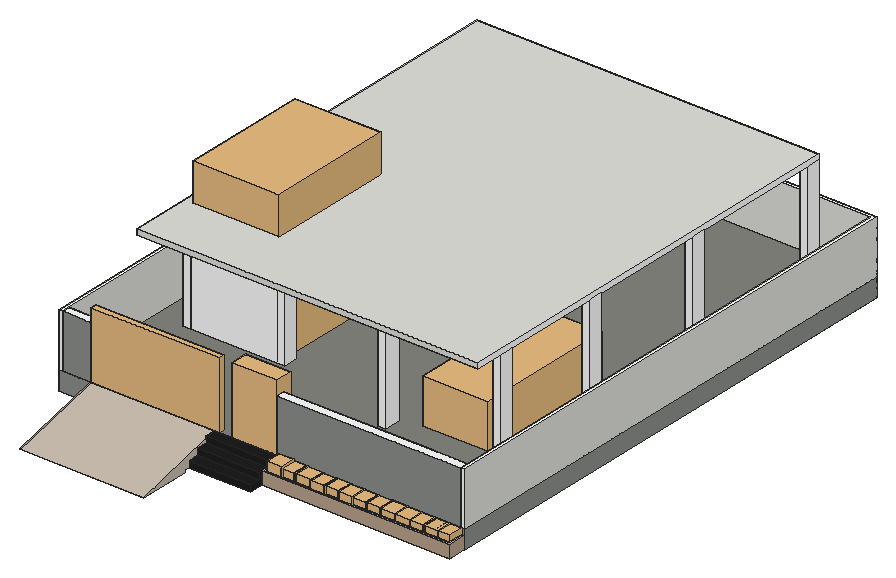
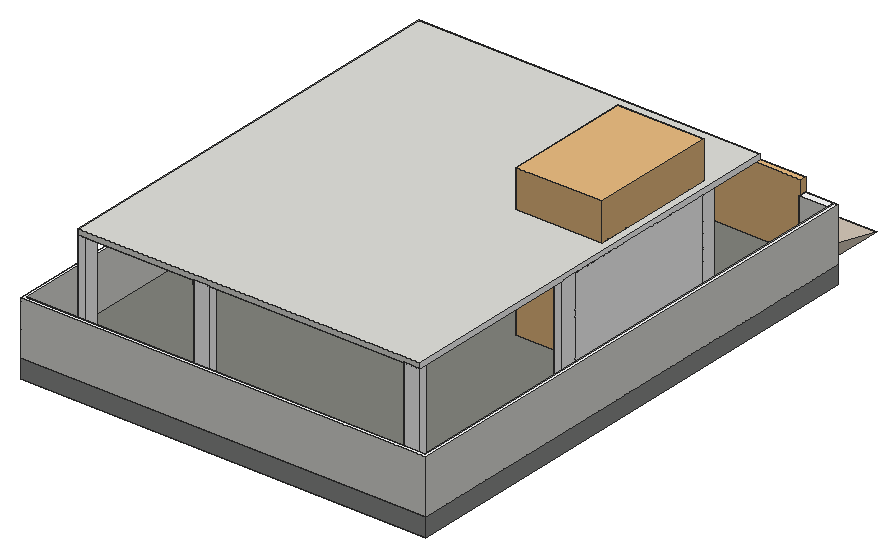
# SketchUp Ruby script. Lengths in inches.
U = 1.inch
M = Sketchup.active_model
def pt(a) = Geom::Point3d.new(a.map { |v| v * U })
def face(e, loops, mat)
  f = e.add_face(loops[0].map { |a| pt(a) })
  loops[1..].each { |l| e.add_face(l.map { |a| pt(a) }).erase! }
  f.material = f.back_material = mat if mat
  f
end
# faces: each face lists its corners as indices into pts; further lists are holes
def faces(e, pts, list, mat = nil) = list.each { |f| face(e, (f[0].is_a?(Array) ? f : [f]).map { |l| l.map { |i| pts[i] } }, mat) }
# xy, xz, yz: faces in a plane at the given z, y or x. An outline is a flat list of corners, or four numbers for a rectangle; further outlines are holes
def ring(l) = l.size == 4 ? [[l[0], l[1]], [l[2], l[1]], [l[2], l[3]], [l[0], l[3]]] : l.each_slice(2).to_a
def flat(e, list, mat, &to3) = list.each { |f| face(e, (f[0].is_a?(Array) ? f : [f]).map { |l| ring(l).map { |u, v| to3.(u, v) } }, mat) }
def xy(e, z, list, mat = nil) = flat(e, list, mat) { |x, y| [x, y, z] }
def xz(e, y, list, mat = nil) = flat(e, list, mat) { |x, z| [x, y, z] }
def yz(e, x, list, mat = nil) = flat(e, list, mat) { |y, z| [x, y, z] }
def lines(e, pts, list) = list.each { |a, b| e.add_line(pt(pts[a]), pt(pts[b])) }
# prism: a flat outline (further loops are holes) pulled along v
def prism(e, loops, v, mat = nil)
  f = face(e, loops, mat); d = Geom::Vector3d.new(v.map { |x| x * U })
  f.pushpull(f.normal.samedirection?(d) ? d.length : -d.length)
end
def box(e, o, s, mat = nil) = prism(e, [[o, [o[0] + s[0], o[1], o[2]], [o[0] + s[0], o[1] + s[1], o[2]], [o[0], o[1] + s[1], o[2]]]], [0, 0, s[2]], mat)
def at(x, y, z, deg = 0) = Geom::Transformation.translation(pt([x, y, z])) * Geom::Transformation.rotation(ORIGIN, Z_AXIS, deg.degrees)
def axes(o, x, y, z) = Geom::Transformation.new([*x, 0, *y, 0, *z, 0, *pt(o).to_a, 1])
def part(name) = M.definitions.add(name)
# library, detail: a bought-in or finely detailed component or shape, given as its bounding box
def library(name, o, s) = part(name).tap { |d| box(d.entities, o, s) }
def detail(e, o, s) = box(e.add_group.entities, o, s)
def put(e, d, t, mat = nil) = e.add_instance(d, t).tap { |i| i.material = mat if mat }
def group(e, t, mat = nil) = e.add_group.tap { |g| g.transformation = t; g.material = mat if mat }.entities
root = M.entities
M.materials.add("Bricks Concrete F01 200cm").color = [143, 145, 142]
M.materials.add("Manhattan Creative Coating MD 1125B 26.44cm").color = [255, 255, 255]
M.materials.add("Manhattan Creative Coating ML 1016B 24.75cm\#1").color = [255, 255, 255]
M.materials.add("Marble Beige 23-86 150cm").color = [204, 192, 177]
M.materials.add("Marble Black 01 150cm\#1").color = [31, 31, 31]
M.materials.add("Sand Stones 01 100cm").color = [188, 164, 143]
M.materials.add("Tiles D 90cm\#1").color = [132, 133, 127]
c1 = library("Ruscus aculeatus 005",[-21.47,-22.21,-0.95],[42.93,43.77,33.94])
c2 = library("Car 026",[-43.02,-94.05,-1.1],[86.04,187.94,58.68])
c3 = part("rthnry")
p = [[12508.04,7803.3,0],[12517.04,7803.3,0],[12517.04,7785.3,0],[12508.04,7785.3,0]]
lines(c3.entities,p,[[0,1],[1,2],[2,3],[3,0]])
c4 = part("rtbhynrj")
p = [[12525.73,7803.3,0],[12534.73,7803.3,0],[12534.73,7788.3,0],[12525.73,7788.3,0]]
lines(c4.entities,p,[[0,1],[1,2],[2,3],[3,0]])
c5 = part("bgghgfgygg")
put(c5.entities,c3,at(6603.41,20471.02,0,-90))
put(c5.entities,c3,at(6838.41,20471.02,0,-90))
put(c5.entities,c3,at(26905.76,15548.77,0,180))
put(c5.entities,c3,at(27149.76,15548.77,0,180))
put(c5.entities,c4,at(1967.98,-236.33,0))
put(c5.entities,c3,at(27149.76,15322.27,0,180))
put(c5.entities,c4,at(1862.98,-236.33,0))
put(c5.entities,c4,at(2235.98,159.67,0))
put(c5.entities,c4,at(2235.98,-0.83,0))
put(c5.entities,c4,at(2235.98,-144.83,0))
put(c5.entities,c4,at(2235.98,-269.33,0))
c6 = library("Group\#154",[0,0,0],[96.64,142.7,167.57])
c7 = library("Group\#145",[0,0,0],[50.48,19.23,75.06])
c8 = library("Group\#146",[0,0,0],[111.6,6.36,75.06])
box(root,[280,194.96,0],[9,18,120],"Manhattan Creative Coating ML 1016B 24.75cm\#1")
box(root,[409,194.96,0],[9,15,120],"Manhattan Creative Coating ML 1016B 24.75cm\#1")
box(root,[409,319.46,0],[9,15,120],"Manhattan Creative Coating ML 1016B 24.75cm\#1")
box(root,[409,463.46,0],[9,15,120],"Manhattan Creative Coating ML 1016B 24.75cm\#1")
prism(root,[[[409,638.96,0],[409,629.96,0],[409,623.96,0],[409,623.96,120],[409,638.96,120]]],[9,0,0],"Manhattan Creative Coating ML 1016B 24.75cm\#1")
box(root,[271,629.96,0],[18,9,120],"Manhattan Creative Coating ML 1016B 24.75cm\#1")
box(root,[36,629.96,0],[18,9,120],"Manhattan Creative Coating ML 1016B 24.75cm\#1")
prism(root,[[[45,425.96,0],[45,421.46,0],[36,421.46,0],[36,439.46,0],[45,439.46,0]]],[0,0,120],"Manhattan Creative Coating ML 1016B 24.75cm\#1")
xy(root,-21,[[36,56.96,174,98.96],[174,62.96,244,98.96],[244,78.4,453.4375,98.96]])
xy(root,-14.4375,[[246.84,81.24,450.6,98.96]],"Sand Stones 01 100cm")
xy(root,-14,[[174,62.96,244,74.9]],"Marble Black 01 150cm\#1")
xy(root,-7,[[174,74.9,244,86.93]],"Marble Black 01 150cm\#1")
xy(root,-7,[[244,78.4,453.4375,78.4,453.4375,98.96,450.6,98.96,450.6,81.24,246.84,81.24,246.84,98.96,244,98.96]],"Sand Stones 01 100cm")
xy(root,0,[[36,98.96,48,107.96],[168,98.96,180,107.96],[228,98.96,240,107.96],[240,98.96,244,107.96]])
xy(root,0,[[36,227.96,45,242.96]],"Manhattan Creative Coating ML 1016B 24.75cm\#1")
xy(root,0,[[174,86.93,244,98.96]],"Marble Black 01 150cm\#1")
xy(root,60,[[4,98.96,36,107.96],[244,98.96,450,107.96]],"Manhattan Creative Coating MD 1125B 26.44cm")
xy(root,120,[[36,227.96,45,242.96],[45,227.96,141,229.96],[141,227.96,150,242.96],[280,421.46,289,439.46]],"Manhattan Creative Coating ML 1016B 24.75cm\#1")
xz(root,56.96,[[36,-23.5,174,-21]])
xz(root,62.96,[[174,-21,244,-14]],"Marble Black 01 150cm\#1")
xz(root,74.9,[[174,-14,244,-7]],"Marble Black 01 150cm\#1")
xz(root,78.4,[[244,-21,453.4375,-7]],"Sand Stones 01 100cm")
xz(root,81.24,[[246.84,-14.4375,450.6,-7]],"Sand Stones 01 100cm")
xz(root,86.93,[[174,-7,244,0]],"Marble Black 01 150cm\#1")
xz(root,98.96,[[36,-21,48,0],[48,-21,168,0],[174,-21,244,0],[244,-21,244,-7,246.84,-7,246.84,-14.4375,450.6,-14.4375,450.6,-7,453.4375,-7,453.4375,-21]])
xz(root,98.96,[[4,0,36,60],[244,0,450,60]],"Bricks Concrete F01 200cm")
xz(root,107.96,[[4,0,36,60],[244,0,409,60],[409,0,418,60],[418,0,450,60]])
xz(root,227.96,[[36,0,45,120],[45,0,141,120],[141,0,150,120]],"Manhattan Creative Coating ML 1016B 24.75cm\#1")
xz(root,229.96,[[45,0,141,120]],"Manhattan Creative Coating ML 1016B 24.75cm\#1")
xz(root,242.96,[[36,0,45,120],[141,0,150,120]],"Manhattan Creative Coating ML 1016B 24.75cm\#1")
xz(root,421.46,[[280,0,289,120]],"Manhattan Creative Coating ML 1016B 24.75cm\#1")
xz(root,439.46,[[280,0,284.5,120],[284.5,0,289,120]],"Manhattan Creative Coating ML 1016B 24.75cm\#1")
yz(root,4,[[98.96,0,107.96,60]])
yz(root,36,[[98.96,0,107.96,60]])
yz(root,36,[[227.96,0,242.96,120]],"Manhattan Creative Coating ML 1016B 24.75cm\#1")
yz(root,36,[[56.96,-23.5,0,-23.45,98.96,0,98.96,-21,56.96,-21]],"Marble Beige 23-86 150cm")
yz(root,45,[[227.96,0,229.96,120],[229.96,0,242.96,120]],"Manhattan Creative Coating ML 1016B 24.75cm\#1")
yz(root,141,[[229.96,0,242.96,120]],"Manhattan Creative Coating ML 1016B 24.75cm\#1")
yz(root,150,[[227.96,0,242.96,120]],"Manhattan Creative Coating ML 1016B 24.75cm\#1")
yz(root,174,[[62.96,-21,98.96,-21,98.96,0,86.93,-2.85,86.93,-7,74.9,-7,74.9,-14,62.96,-14],[86.93,-2.85,98.96,0,86.93,0]])
yz(root,174,[[56.96,-23.5,56.96,-21,62.96,-21,62.96,-14,74.9,-14,74.9,-7,86.93,-7,86.93,-2.85,0,-23.45]],"Marble Beige 23-86 150cm")
yz(root,244,[[78.4,-21,98.96,-7],[98.96,0,107.96,60]])
yz(root,244,[[62.96,-21,78.4,-21,78.4,-7,74.9,-7,74.9,-14,62.96,-14],[86.93,-7,98.96,0]],"Marble Black 01 150cm\#1")
yz(root,246.84,[[81.24,-14.4375,98.96,-7]],"Sand Stones 01 100cm")
yz(root,280,[[421.46,0,439.46,120]],"Manhattan Creative Coating ML 1016B 24.75cm\#1")
yz(root,289,[[421.46,0,439.46,120]],"Manhattan Creative Coating ML 1016B 24.75cm\#1")
yz(root,450,[[98.96,0,107.96,60]])
yz(root,450.6,[[81.24,-14.4375,98.96,-7]])
yz(root,453.4375,[[78.4,-21,98.96,-7]],"Sand Stones 01 100cm")
p = [[36,98.96,0],[36,0,-23.45],[174,0,-23.45],[174,86.93,-2.85],[174,98.96,0],[168,98.96,0],
  [48,98.96,0],[36,56.96,-23.5],[174,56.96,-23.5],[45,268.96,0],[45,242.96,0],[45,283.54,0],
  [45,278.96,0],[45,368.96,0],[45,421.46,0],[45,358.96,0],[102,368.96,0],[102,358.96,0],
  [141,358.96,0],[84,278.96,70],[93.1875,278.96,70],[102.375,278.96,70],[93.1875,269.27,70]]
faces(root,p,[[0,1,2,3,4,5,6]],"Marble Beige 23-86 150cm")
faces(root,p,[[2,1,7,8]])
lines(root,p,[[9,10],[11,12],[13,14],[15,11],[13,15],[16,17],[17,18],[19,20],[20,21],[20,22]])
g1 = group(root,at(36,98.96,-6))
xy(g1,-15,[[-36,0,418,576]])
xy(g1,6,[[-36,0,418,576]],"Tiles D 90cm\#1")
xz(g1,0,[[-36,-15,418,6]],"Bricks Concrete F01 200cm")
xz(g1,576,[[-36,-15,418,6]],"Bricks Concrete F01 200cm")
yz(g1,-36,[[0,-15,576,6]],"Bricks Concrete F01 200cm")
yz(g1,418,[[0,-15,576,6]],"Bricks Concrete F01 200cm")
put(root,c1,axes([365.7,90.55,-17.24],[0.39,0,0],[0,0.39,0],[0,0,0.53451]))
put(root,c1,axes([255.39,89.9,-13.94],[0.39,0,0],[0,0.39,0],[0,0,0.5187]))
put(root,c1,axes([334.22,89.83,-14.01],[0.39,0,0],[0,0.39,0],[0,0,0.44996]))
put(root,c1,axes([304.02,89.66,-14],[0.39,0,0],[0,0.39,0],[0,0,0.45584]))
put(root,c1,axes([381.84,90.37,-14.02],[0.39,0,0],[0,0.39,0],[0,0,0.43704]))
put(root,c1,axes([414.59,90.37,-14.03],[0.39,0,0],[0,0.39,0],[0,0,0.42584]))
put(root,c1,axes([286.66,90.55,-14],[0.4602,0,0],[0,0.39,0],[0,0,0.46248]))
put(root,c1,axes([350.12,90.01,-14.01],[0.39,0,0],[0,0.39,0],[0,0,0.44416]))
put(root,c1,axes([429.53,90.37,-14.03],[0.39,0,0],[0,0.39,0],[0,0,0.42584]))
put(root,c1,axes([398.21,90.37,-14.03],[0.39,0,0],[0,0.39,0],[0,0,0.4314]))
put(root,c1,axes([270.67,90.55,-13.99],[0.39,0,0],[0,0.39,0],[0,0,0.47001]))
put(root,c1,axes([319.02,90.55,-14],[0.39,0,0],[0,0.39,0],[0,0,0.45584]))
put(root,c1,axes([442.23,90.55,-14.04],[0.39,0,0],[0,0.39,0],[0,0,0.42035]))
put(root,c2,axes([346.91,299.51,0.9375],[0.8494,0,0],[0,0.8494,0],[0,0,0.8494]))
put(root,c5,at(-14352.71,-7324.01,0))
g2 = group(root,at(36,242.96,0))
xy(g2,0,[[0,0,9,178.5]])
xy(g2,120,[[0,0,9,178.5]])
xz(g2,0,[[0,0,9,120]])
xz(g2,178.5,[[0,0,9,120]])
yz(g2,0,[[0,0,178.5,120]],"Manhattan Creative Coating ML 1016B 24.75cm\#1")
yz(g2,9,[[0,0,178.5,120]])
put(root,c6,at(45,229.96,0))
put(root,c7,at(193.52,98.96,0))
put(root,c8,axes([36,98.96,0],[1.29037,0,0],[0,1,0],[0,0,1]))
g3 = group(root,at(0,98.96,0))
xy(g3,0,[[0,0,0,576,454,576,454,0,450,0,450,572,4,572,4,0]])
xy(g3,60,[[0,0,4,0,4,572,450,572,450,0,454,0,454,576,0,576]],"Manhattan Creative Coating MD 1125B 26.44cm")
xz(g3,0,[[0,0,4,60],[450,0,454,60]],"Manhattan Creative Coating MD 1125B 26.44cm")
xz(g3,572,[[4,0,450,60]])
xz(g3,576,[[0,0,454,60]])
yz(g3,0,[[0,0,576,60]])
yz(g3,4,[[0,0,572,60]])
yz(g3,450,[[0,0,572,60]])
yz(g3,454,[[0,0,576,60]])
g4 = group(root,at(36,98.96,120))
xy(g4,0,[[[0,63.75,382,540],[9,131,105,270]]])
xy(g4,6,[[[0,63.75,382,540],[9,131,105,270]]])
xz(g4,63.75,[[0,0,382,6]])
xz(g4,131,[[9,0,105,6]])
xz(g4,270,[[9,0,105,6]])
xz(g4,540,[[0,0,382,6]])
yz(g4,0,[[63.75,0,540,6]],"Manhattan Creative Coating MD 1125B 26.44cm")
yz(g4,9,[[131,0,270,6]])
yz(g4,105,[[131,0,270,6]])
yz(g4,382,[[63.75,0,540,6]],"Manhattan Creative Coating MD 1125B 26.44cm")
